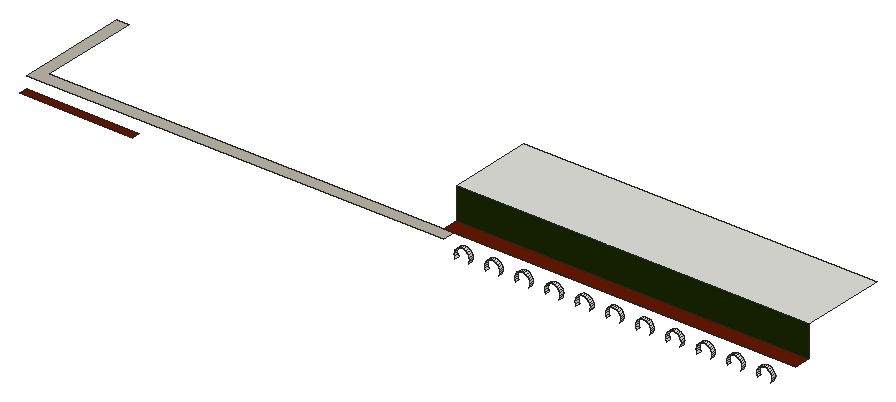
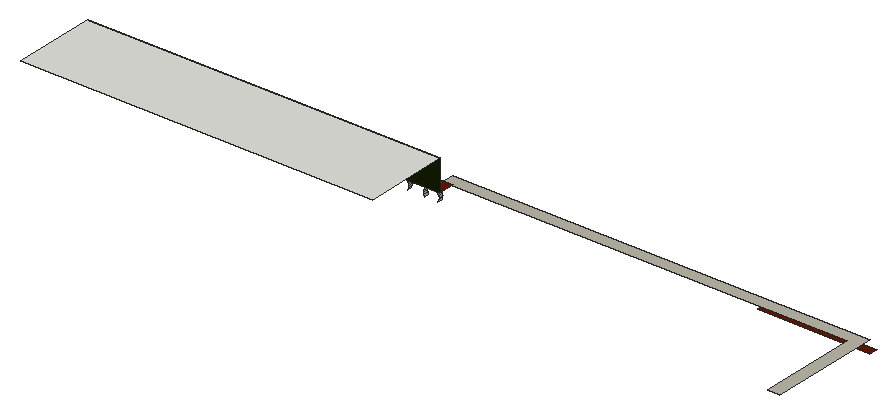
# SketchUp Ruby script. Lengths in inches.
U = 1.inch
M = Sketchup.active_model
def pt(a) = Geom::Point3d.new(a.map { |v| v * U })
def face(e, loops, mat)
  f = e.add_face(loops[0].map { |a| pt(a) })
  loops[1..].each { |l| e.add_face(l.map { |a| pt(a) }).erase! }
  f.material = f.back_material = mat if mat
  f
end
# faces: each face lists its corners as indices into pts; further lists are holes
def faces(e, pts, list, mat = nil) = list.each { |f| face(e, (f[0].is_a?(Array) ? f : [f]).map { |l| l.map { |i| pts[i] } }, mat) }
# xy, xz, yz: faces in a plane at the given z, y or x. An outline is a flat list of corners, or four numbers for a rectangle; further outlines are holes
def ring(l) = l.size == 4 ? [[l[0], l[1]], [l[2], l[1]], [l[2], l[3]], [l[0], l[3]]] : l.each_slice(2).to_a
def flat(e, list, mat, &to3) = list.each { |f| face(e, (f[0].is_a?(Array) ? f : [f]).map { |l| ring(l).map { |u, v| to3.(u, v) } }, mat) }
def xy(e, z, list, mat = nil) = flat(e, list, mat) { |x, y| [x, y, z] }
def xz(e, y, list, mat = nil) = flat(e, list, mat) { |x, z| [x, y, z] }
def yz(e, x, list, mat = nil) = flat(e, list, mat) { |y, z| [x, y, z] }
def lines(e, pts, list) = list.each { |a, b| e.add_line(pt(pts[a]), pt(pts[b])) }
# prism: a flat outline (further loops are holes) pulled along v
def prism(e, loops, v, mat = nil)
  f = face(e, loops, mat); d = Geom::Vector3d.new(v.map { |x| x * U })
  f.pushpull(f.normal.samedirection?(d) ? d.length : -d.length)
end
def box(e, o, s, mat = nil) = prism(e, [[o, [o[0] + s[0], o[1], o[2]], [o[0] + s[0], o[1] + s[1], o[2]], [o[0], o[1] + s[1], o[2]]]], [0, 0, s[2]], mat)
def at(x, y, z, deg = 0) = Geom::Transformation.translation(pt([x, y, z])) * Geom::Transformation.rotation(ORIGIN, Z_AXIS, deg.degrees)
def axes(o, x, y, z) = Geom::Transformation.new([*x, 0, *y, 0, *z, 0, *pt(o).to_a, 1])
def part(name) = M.definitions.add(name)
# library, detail: a bought-in or finely detailed component or shape, given as its bounding box
def library(name, o, s) = part(name).tap { |d| box(d.entities, o, s) }
def detail(e, o, s) = box(e.add_group.entities, o, s)
def put(e, d, t, mat = nil) = e.add_instance(d, t).tap { |i| i.material = mat if mat }
def group(e, t, mat = nil) = e.add_group.tap { |g| g.transformation = t; g.material = mat if mat }.entities
root = M.entities
M.materials.add("[0060_GrassGreen]").color = [27, 40, 2]
M.materials.add("[Color B08]").color = [102, 25, 0]
M.materials.add("[Formica Graystone]1").color = [186, 182, 168]
xy(root,518.76,[[3.53,171.0625,87.4,177.0625]],"[Color B08]")
xy(root,528,[[3.53,177.0625,314.59,177.0625,314.59,186.0625,12.53,186.0625,12.53,261.0625,3.53,261.0625]],"[Formica Graystone]1")
xy(root,528.49,[[307.22,186.0625,569.78,198.0625]],"[Color B08]")
xy(root,551.875,[[307.22,198.0625,569.78,261.0625]])
xz(root,198.0625,[[307.22,528.49,569.78,551.875]],"[0060_GrassGreen]")
p = [[317.56,186.0625,515],[318.13,186.0625,513.61],[318.13,183.0625,513.61],[317.56,183.0625,515],[328.09,186.0625,513.61],[328.66,186.0625,515],
  [328.66,183.0625,515],[328.09,183.0625,513.61],[340.12,186.0625,515],[340.69,186.0625,513.61],[340.69,183.0625,513.61],[340.12,183.0625,515],
  [350.65,186.0625,513.61],[351.23,186.0625,515],[351.23,183.0625,515],[350.65,183.0625,513.61],[362.68,186.0625,515],[363.26,186.0625,513.61],
  [363.26,183.0625,513.61],[362.68,183.0625,515],[373.22,186.0625,513.61],[373.79,186.0625,515],[373.79,183.0625,515],[373.22,183.0625,513.61],
  [385.24,186.0625,515],[385.82,186.0625,513.61],[385.82,183.0625,513.61],[385.24,183.0625,515],[395.78,186.0625,513.61],[396.35,186.0625,515],
  [396.35,183.0625,515],[395.78,183.0625,513.61],[407.81,186.0625,515],[408.38,186.0625,513.61],[408.38,183.0625,513.61],[407.81,183.0625,515],
  [418.34,186.0625,513.61],[418.91,186.0625,515],[418.91,183.0625,515],[418.34,183.0625,513.61],[430.37,186.0625,515],[430.94,186.0625,513.61],
  [430.94,183.0625,513.61],[430.37,183.0625,515],[440.9,186.0625,513.61],[441.48,186.0625,515],[441.48,183.0625,515],[440.9,183.0625,513.61],
  [452.93,186.0625,515],[453.51,186.0625,513.61],[453.51,183.0625,513.61],[452.93,183.0625,515],[463.47,186.0625,513.61],[464.04,186.0625,515],
  [464.04,183.0625,515],[463.47,183.0625,513.61],[475.49,186.0625,515],[476.07,186.0625,513.61],[476.07,183.0625,513.61],[475.49,183.0625,515],
  [486.03,186.0625,513.61],[486.6,186.0625,515],[486.6,183.0625,515],[486.03,183.0625,513.61],[498.06,186.0625,515],[498.63,186.0625,513.61],
  [498.63,183.0625,513.61],[498.06,183.0625,515],[508.59,186.0625,513.61],[509.16,186.0625,515],[509.16,183.0625,515],[508.59,183.0625,513.61],
  [520.62,186.0625,515],[521.19,186.0625,513.61],[521.19,183.0625,513.61],[520.62,183.0625,515],[531.15,186.0625,513.61],[531.73,186.0625,515],
  [531.73,183.0625,515],[531.15,183.0625,513.61],[543.18,186.0625,515],[543.76,186.0625,513.61],[543.76,183.0625,513.61],[543.18,183.0625,515],
  [553.72,186.0625,513.61],[554.29,186.0625,515],[554.29,183.0625,515],[553.72,183.0625,513.61],[317.36,186.0625,516.49],[317.36,183.0625,516.49],
  [328.86,186.0625,516.49],[328.86,183.0625,516.49],[339.92,186.0625,516.49],[339.92,183.0625,516.49],[351.42,186.0625,516.49],[351.42,183.0625,516.49],
  [362.49,186.0625,516.49],[362.49,183.0625,516.49],[373.99,186.0625,516.49],[373.99,183.0625,516.49],[385.05,186.0625,516.49],[385.05,183.0625,516.49],
  [396.55,186.0625,516.49],[396.55,183.0625,516.49],[407.61,186.0625,516.49],[407.61,183.0625,516.49],[419.11,186.0625,516.49],[419.11,183.0625,516.49],
  [430.17,186.0625,516.49],[430.17,183.0625,516.49],[441.67,186.0625,516.49],[441.67,183.0625,516.49],[452.74,186.0625,516.49],[452.74,183.0625,516.49],
  [464.24,186.0625,516.49],[464.24,183.0625,516.49],[475.3,186.0625,516.49],[475.3,183.0625,516.49],[486.8,186.0625,516.49],[486.8,183.0625,516.49],
  [497.86,186.0625,516.49],[497.86,183.0625,516.49],[509.36,186.0625,516.49],[509.36,183.0625,516.49],[520.42,186.0625,516.49],[520.42,183.0625,516.49],
  [531.92,186.0625,516.49],[531.92,183.0625,516.49],[542.99,186.0625,516.49],[542.99,183.0625,516.49],[554.49,186.0625,516.49],[554.49,183.0625,516.49],
  [317.56,186.0625,517.97],[317.56,183.0625,517.97],[328.66,186.0625,517.97],[328.66,183.0625,517.97],[340.12,186.0625,517.97],[340.12,183.0625,517.97],
  [351.23,186.0625,517.97],[351.23,183.0625,517.97],[362.68,186.0625,517.97],[362.68,183.0625,517.97],[373.79,186.0625,517.97],[373.79,183.0625,517.97],
  [385.24,186.0625,517.97],[385.24,183.0625,517.97],[396.35,186.0625,517.97],[396.35,183.0625,517.97],[407.81,186.0625,517.97],[407.81,183.0625,517.97],
  [418.91,186.0625,517.97],[418.91,183.0625,517.97],[430.37,186.0625,517.97],[430.37,183.0625,517.97],[441.48,186.0625,517.97],[441.48,183.0625,517.97],
  [452.93,186.0625,517.97],[452.93,183.0625,517.97],[464.04,186.0625,517.97],[464.04,183.0625,517.97],[475.49,186.0625,517.97],[475.49,183.0625,517.97],
  [486.6,186.0625,517.97],[486.6,183.0625,517.97],[498.06,186.0625,517.97],[498.06,183.0625,517.97],[509.16,186.0625,517.97],[509.16,183.0625,517.97],
  [520.62,186.0625,517.97],[520.62,183.0625,517.97],[531.73,186.0625,517.97],[531.73,183.0625,517.97],[543.18,186.0625,517.97],[543.18,183.0625,517.97],
  [554.29,186.0625,517.97],[554.29,183.0625,517.97],[318.13,186.0625,519.36],[318.13,183.0625,519.36],[328.09,186.0625,519.36],[328.09,183.0625,519.36],
  [340.69,186.0625,519.36],[340.69,183.0625,519.36],[350.65,186.0625,519.36],[350.65,183.0625,519.36],[363.26,186.0625,519.36],[363.26,183.0625,519.36],
  [373.22,186.0625,519.36],[373.22,183.0625,519.36],[385.82,186.0625,519.36],[385.82,183.0625,519.36],[395.78,186.0625,519.36],[395.78,183.0625,519.36],
  [408.38,186.0625,519.36],[408.38,183.0625,519.36],[418.34,186.0625,519.36],[418.34,183.0625,519.36],[430.94,186.0625,519.36],[430.94,183.0625,519.36],
  [440.9,186.0625,519.36],[440.9,183.0625,519.36],[453.51,186.0625,519.36],[453.51,183.0625,519.36],[463.47,186.0625,519.36],[463.47,183.0625,519.36],
  [476.07,186.0625,519.36],[476.07,183.0625,519.36],[486.03,186.0625,519.36],[486.03,183.0625,519.36],[498.63,186.0625,519.36],[498.63,183.0625,519.36],
  [508.59,186.0625,519.36],[508.59,183.0625,519.36],[521.19,186.0625,519.36],[521.19,183.0625,519.36],[531.15,186.0625,519.36],[531.15,183.0625,519.36],
  [543.76,186.0625,519.36],[543.76,183.0625,519.36],[553.72,186.0625,519.36],[553.72,183.0625,519.36],[319.04,186.0625,520.55],[319.04,183.0625,520.55],
  [327.18,186.0625,520.55],[327.18,183.0625,520.55],[341.61,186.0625,520.55],[341.61,183.0625,520.55],[349.74,186.0625,520.55],[349.74,183.0625,520.55],
  [364.17,186.0625,520.55],[364.17,183.0625,520.55],[372.3,186.0625,520.55],[372.3,183.0625,520.55],[386.73,186.0625,520.55],[386.73,183.0625,520.55],
  [394.86,186.0625,520.55],[394.86,183.0625,520.55],[409.29,186.0625,520.55],[409.29,183.0625,520.55],[417.43,186.0625,520.55],[417.43,183.0625,520.55],
  [431.86,186.0625,520.55],[431.86,183.0625,520.55],[439.99,186.0625,520.55],[439.99,183.0625,520.55],[454.42,186.0625,520.55],[454.42,183.0625,520.55],
  [462.55,186.0625,520.55],[462.55,183.0625,520.55],[476.98,186.0625,520.55],[476.98,183.0625,520.55],[485.11,186.0625,520.55],[485.11,183.0625,520.55],
  [499.54,186.0625,520.55],[499.54,183.0625,520.55],[507.68,186.0625,520.55],[507.68,183.0625,520.55],[522.11,186.0625,520.55],[522.11,183.0625,520.55],
  [530.24,186.0625,520.55],[530.24,183.0625,520.55],[544.67,186.0625,520.55],[544.67,183.0625,520.55],[552.8,186.0625,520.55],[552.8,183.0625,520.55],
  [320.24,186.0625,521.46],[320.24,183.0625,521.46],[325.99,186.0625,521.46],[325.99,183.0625,521.46],[342.8,186.0625,521.46],[342.8,183.0625,521.46],
  [348.55,186.0625,521.46],[348.55,183.0625,521.46],[365.36,186.0625,521.46],[365.36,183.0625,521.46],[371.11,186.0625,521.46],[371.11,183.0625,521.46],
  [387.92,186.0625,521.46],[387.92,183.0625,521.46],[393.67,186.0625,521.46],[393.67,183.0625,521.46],[410.49,186.0625,521.46],[410.49,183.0625,521.46],
  [416.24,186.0625,521.46],[416.24,183.0625,521.46],[433.05,186.0625,521.46],[433.05,183.0625,521.46],[438.8,186.0625,521.46],[438.8,183.0625,521.46],
  [455.61,186.0625,521.46],[455.61,183.0625,521.46],[461.36,186.0625,521.46],[461.36,183.0625,521.46],[478.17,186.0625,521.46],[478.17,183.0625,521.46],
  [483.92,186.0625,521.46],[483.92,183.0625,521.46],[500.74,186.0625,521.46],[500.74,183.0625,521.46],[506.49,186.0625,521.46],[506.49,183.0625,521.46],
  [523.3,186.0625,521.46],[523.3,183.0625,521.46],[529.05,186.0625,521.46],[529.05,183.0625,521.46],[545.86,186.0625,521.46],[545.86,183.0625,521.46],
  [551.61,186.0625,521.46],[551.61,183.0625,521.46],[321.62,186.0625,522.04],[321.62,183.0625,522.04],[324.6,186.0625,522.04],[324.6,183.0625,522.04],
  [344.19,186.0625,522.04],[344.19,183.0625,522.04],[347.16,186.0625,522.04],[347.16,183.0625,522.04],[366.75,186.0625,522.04],[366.75,183.0625,522.04],
  [369.72,186.0625,522.04],[369.72,183.0625,522.04],[389.31,186.0625,522.04],[389.31,183.0625,522.04],[392.29,186.0625,522.04],[392.29,183.0625,522.04],
  [411.87,186.0625,522.04],[411.87,183.0625,522.04],[414.85,186.0625,522.04],[414.85,183.0625,522.04],[434.44,186.0625,522.04],[434.44,183.0625,522.04],
  [437.41,186.0625,522.04],[437.41,183.0625,522.04],[457,186.0625,522.04],[457,183.0625,522.04],[459.97,186.0625,522.04],[459.97,183.0625,522.04],
  [479.56,186.0625,522.04],[479.56,183.0625,522.04],[482.54,186.0625,522.04],[482.54,183.0625,522.04],[502.12,186.0625,522.04],[502.12,183.0625,522.04],
  [505.1,186.0625,522.04],[505.1,183.0625,522.04],[524.69,186.0625,522.04],[524.69,183.0625,522.04],[527.66,186.0625,522.04],[527.66,183.0625,522.04],
  [547.25,186.0625,522.04],[547.25,183.0625,522.04],[550.22,186.0625,522.04],[550.22,183.0625,522.04],[323.11,186.0625,522.24],[323.11,183.0625,522.24],
  [345.67,186.0625,522.24],[345.67,183.0625,522.24],[368.24,186.0625,522.24],[368.24,183.0625,522.24],[390.8,186.0625,522.24],[390.8,183.0625,522.24],
  [413.36,186.0625,522.24],[413.36,183.0625,522.24],[435.92,186.0625,522.24],[435.92,183.0625,522.24],[458.49,186.0625,522.24],[458.49,183.0625,522.24],
  [481.05,186.0625,522.24],[481.05,183.0625,522.24],[503.61,186.0625,522.24],[503.61,183.0625,522.24],[526.17,186.0625,522.24],[526.17,183.0625,522.24],
  [548.74,186.0625,522.24],[548.74,183.0625,522.24]]
faces(root,p,[[0,1,2,3],[4,5,6,7],[8,9,10,11],[12,13,14,15],[16,17,18,19],[20,21,22,23],[24,25,26,27],[28,29,30,31],
  [32,33,34,35],[36,37,38,39],[40,41,42,43],[44,45,46,47],[48,49,50,51],[52,53,54,55],[56,57,58,59],[60,61,62,63],
  [64,65,66,67],[68,69,70,71],[72,73,74,75],[76,77,78,79],[80,81,82,83],[84,85,86,87],[88,0,3,89],[5,90,91,6],
  [92,8,11,93],[13,94,95,14],[96,16,19,97],[21,98,99,22],[100,24,27,101],[29,102,103,30],[104,32,35,105],[37,106,107,38],
  [108,40,43,109],[45,110,111,46],[112,48,51,113],[53,114,115,54],[116,56,59,117],[61,118,119,62],[120,64,67,121],[69,122,123,70],
  [124,72,75,125],[77,126,127,78],[128,80,83,129],[85,130,131,86],[132,88,89,133],[90,134,135,91],[136,92,93,137],[94,138,139,95],
  [140,96,97,141],[98,142,143,99],[144,100,101,145],[102,146,147,103],[148,104,105,149],[106,150,151,107],[152,108,109,153],[110,154,155,111],
  [156,112,113,157],[114,158,159,115],[160,116,117,161],[118,162,163,119],[164,120,121,165],[122,166,167,123],[168,124,125,169],[126,170,171,127],
  [172,128,129,173],[130,174,175,131],[176,132,133,177],[134,178,179,135],[180,136,137,181],[138,182,183,139],[184,140,141,185],[142,186,187,143],
  [188,144,145,189],[146,190,191,147],[192,148,149,193],[150,194,195,151],[196,152,153,197],[154,198,199,155],[200,156,157,201],[158,202,203,159],
  [204,160,161,205],[162,206,207,163],[208,164,165,209],[166,210,211,167],[212,168,169,213],[170,214,215,171],[216,172,173,217],[174,218,219,175],
  [220,176,177,221],[178,222,223,179],[224,180,181,225],[182,226,227,183],[228,184,185,229],[186,230,231,187],[232,188,189,233],[190,234,235,191],
  [236,192,193,237],[194,238,239,195],[240,196,197,241],[198,242,243,199],[244,200,201,245],[202,246,247,203],[248,204,205,249],[206,250,251,207],
  [252,208,209,253],[210,254,255,211],[256,212,213,257],[214,258,259,215],[260,216,217,261],[218,262,263,219],[264,220,221,265],[222,266,267,223],
  [268,224,225,269],[226,270,271,227],[272,228,229,273],[230,274,275,231],[276,232,233,277],[234,278,279,235],[280,236,237,281],[238,282,283,239],
  [284,240,241,285],[242,286,287,243],[288,244,245,289],[246,290,291,247],[292,248,249,293],[250,294,295,251],[296,252,253,297],[254,298,299,255],
  [300,256,257,301],[258,302,303,259],[304,260,261,305],[262,306,307,263],[308,264,265,309],[266,310,311,267],[312,268,269,313],[270,314,315,271],
  [316,272,273,317],[274,318,319,275],[320,276,277,321],[278,322,323,279],[324,280,281,325],[282,326,327,283],[328,284,285,329],[286,330,331,287],
  [332,288,289,333],[290,334,335,291],[336,292,293,337],[294,338,339,295],[340,296,297,341],[298,342,343,299],[344,300,301,345],[302,346,347,303],
  [348,304,305,349],[306,350,351,307],[352,308,309,353],[310,352,353,311],[354,312,313,355],[314,354,355,315],[356,316,317,357],[318,356,357,319],
  [358,320,321,359],[322,358,359,323],[360,324,325,361],[326,360,361,327],[362,328,329,363],[330,362,363,331],[364,332,333,365],[334,364,365,335],
  [366,336,337,367],[338,366,367,339],[368,340,341,369],[342,368,369,343],[370,344,345,371],[346,370,371,347],[372,348,349,373],[350,372,373,351]])
